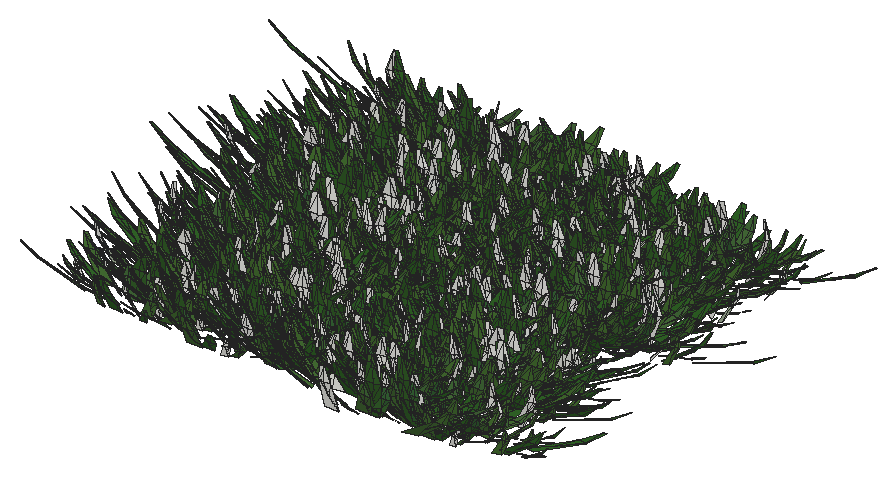
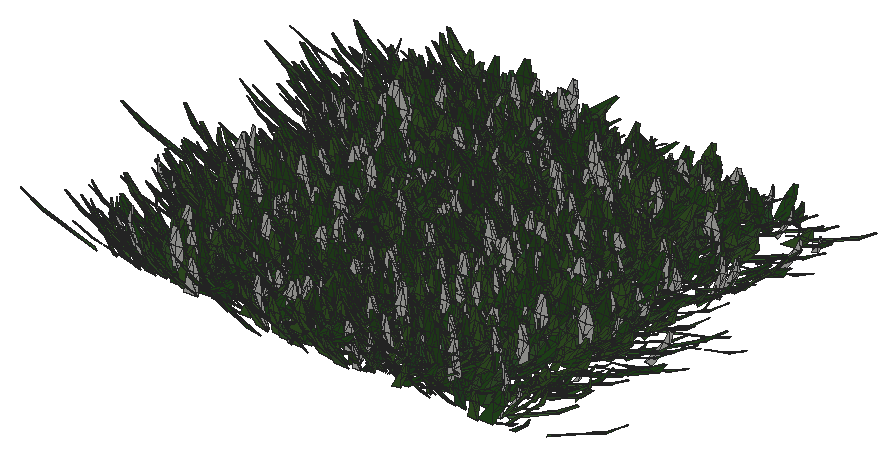
# SketchUp Ruby script. Lengths in inches.
U = 1.inch
M = Sketchup.active_model
def pt(a) = Geom::Point3d.new(a.map { |v| v * U })
def face(e, loops, mat)
  f = e.add_face(loops[0].map { |a| pt(a) })
  loops[1..].each { |l| e.add_face(l.map { |a| pt(a) }).erase! }
  f.material = f.back_material = mat if mat
  f
end
# faces: each face lists its corners as indices into pts; further lists are holes
def faces(e, pts, list, mat = nil) = list.each { |f| face(e, (f[0].is_a?(Array) ? f : [f]).map { |l| l.map { |i| pts[i] } }, mat) }
# xy, xz, yz: faces in a plane at the given z, y or x. An outline is a flat list of corners, or four numbers for a rectangle; further outlines are holes
def ring(l) = l.size == 4 ? [[l[0], l[1]], [l[2], l[1]], [l[2], l[3]], [l[0], l[3]]] : l.each_slice(2).to_a
def flat(e, list, mat, &to3) = list.each { |f| face(e, (f[0].is_a?(Array) ? f : [f]).map { |l| ring(l).map { |u, v| to3.(u, v) } }, mat) }
def xy(e, z, list, mat = nil) = flat(e, list, mat) { |x, y| [x, y, z] }
def xz(e, y, list, mat = nil) = flat(e, list, mat) { |x, z| [x, y, z] }
def yz(e, x, list, mat = nil) = flat(e, list, mat) { |y, z| [x, y, z] }
def lines(e, pts, list) = list.each { |a, b| e.add_line(pt(pts[a]), pt(pts[b])) }
# prism: a flat outline (further loops are holes) pulled along v
def prism(e, loops, v, mat = nil)
  f = face(e, loops, mat); d = Geom::Vector3d.new(v.map { |x| x * U })
  f.pushpull(f.normal.samedirection?(d) ? d.length : -d.length)
end
def box(e, o, s, mat = nil) = prism(e, [[o, [o[0] + s[0], o[1], o[2]], [o[0] + s[0], o[1] + s[1], o[2]], [o[0], o[1] + s[1], o[2]]]], [0, 0, s[2]], mat)
def at(x, y, z, deg = 0) = Geom::Transformation.translation(pt([x, y, z])) * Geom::Transformation.rotation(ORIGIN, Z_AXIS, deg.degrees)
def axes(o, x, y, z) = Geom::Transformation.new([*x, 0, *y, 0, *z, 0, *pt(o).to_a, 1])
def part(name) = M.definitions.add(name)
# library, detail: a bought-in or finely detailed component or shape, given as its bounding box
def library(name, o, s) = part(name).tap { |d| box(d.entities, o, s) }
def detail(e, o, s) = box(e.add_group.entities, o, s)
def put(e, d, t, mat = nil) = e.add_instance(d, t).tap { |i| i.material = mat if mat }
def group(e, t, mat = nil) = e.add_group.tap { |g| g.transformation = t; g.material = mat if mat }.entities
root = M.entities
M.materials.add("Material10").color = [48, 100, 38]
M.materials.add("Material3").color = [68, 110, 58]
M.materials.add("Material4").color = [48, 90, 38]
M.materials.add("Material5").color = [68, 110, 48]
M.materials.add("Material6").color = [48, 90, 48]
M.materials.add("Material7").color = [58, 110, 58]
M.materials.add("Material8").color = [58, 90, 38]
M.materials.add("Material9").color = [68, 100, 58]
c1 = part("grass00")
p = [[-0.6875,0.15,0],[-0.56,0.08,5.52],[-0.04,0.03,2.76],[0.48,-0.02,0],[0.35,-0.02,5.52],[-0.1,-0.14,5.52],
  [-0.12,0.65,8.37],[-0.42,0.65,8.37]]
faces(c1.entities,p,[[0,1,2,3],[3,2,4],[1,5,2],[5,4,2],[1,6,5],[4,5,6],[7,6,1]])
c2 = part("Group16\#1")
put(c2.entities,c1,axes([1.44,-0.61,-0.01],[0.05352,0.12609,0],[-0.10704,0.04543,0.07239],[0.06664,-0.02828,0.11628]),"Material6")
put(c2.entities,c1,axes([0.76,-0.15,-0.01],[0.04676,0.24062,0],[-0.23162,0.04501,0.06642],[0.0652,-0.01267,0.23595]),"Material3")
put(c2.entities,c1,axes([0.79,0.01,-0.01],[-0.00606,0.34651,0],[-0.34381,-0.00602,0.0432],[0.04319,0.00076,0.34386]))
put(c2.entities,c1,axes([1,0.23,-0.01],[-0.07192,0.31144,0],[-0.28722,-0.06632,0.1236],[0.12043,0.02781,0.29478]),"Material5")
put(c2.entities,c1,axes([1.66,0.77,-0.01],[-0.13828,0.29651,0],[-0.21551,-0.1005,0.22471],[0.20365,0.09498,0.23779]),"Material10")
put(c2.entities,c1,axes([0.6875,0.52,-0.01],[-0.18126,0.24051,0],[-0.22746,-0.17142,0.09788],[0.07817,0.05891,0.28481]),"Material5")
put(c2.entities,c1,axes([0.68,0.78,-0.01],[-0.215,0.18688,0],[-0.12385,-0.14248,0.21334],[0.13995,0.16101,0.18878]),"Material3")
put(c2.entities,c1,axes([0.56,1,-0.01],[-0.13756,0.07624,0],[-0.06159,-0.11112,0.0927],[0.04494,0.08108,0.12705]),"Material5")
put(c2.entities,c1,axes([0.2,0.64,-0.01],[-0.23729,0.07254,0],[-0.05711,-0.18681,0.153],[0.04473,0.14632,0.19535]),"Material10")
put(c2.entities,c1,axes([0.0625,0.72,-0.01],[-0.28874,0.02525,0],[-0.02179,-0.24916,0.14647],[0.01276,0.14591,0.25012]),"Material3")
put(c2.entities,c1,axes([-0.08,0.62,-0.01],[-0.34089,-0.04187,0],[0.03255,-0.26504,0.216],[-0.02633,0.21439,0.26703]),"Material10")
put(c2.entities,c1,axes([-0.34,0.98,-0.01],[-0.14314,-0.0493,0],[0.04397,-0.12769,0.06843],[-0.02228,0.0647,0.13505]),"Material10")
put(c2.entities,c1,axes([-0.87,1.45,-0.01],[-0.23488,-0.14114,0],[0.13761,-0.22901,0.06087],[-0.03135,0.05217,0.26717]))
put(c2.entities,c1,axes([-0.72,0.77,-0.01],[-0.14208,-0.13251,0],[0.07209,-0.0773,0.16301],[-0.11118,0.11922,0.1057]),"Material10")
put(c2.entities,c1,axes([-0.62,0.43,-0.01],[-0.14845,-0.21203,0],[0.18654,-0.13061,0.12304],[-0.10079,0.07057,0.22772]),"Material3")
put(c2.entities,c1,axes([-0.68,0.29,-0.01],[-0.13639,-0.32136,0],[0.31723,-0.13464,0.05579],[-0.05136,0.0218,0.34462]),"Material4")
put(c2.entities,c1,axes([-0.64,0.125,-0.01],[-0.0458,-0.23569,0],[0.22124,-0.043,0.08276],[-0.08124,0.01579,0.22538]),"Material7")
put(c2.entities,c1,axes([-1.6,-0.03,-0.01],[0.00576,-0.32897,0],[0.27526,0.00482,0.18018],[-0.18015,-0.00315,0.2753]),"Material5")
put(c2.entities,c1,axes([-1.36,-0.31,-0.01],[0.05718,-0.24765,0],[0.18172,0.04196,0.17267],[-0.16825,-0.03885,0.1865]),"Material10")
put(c2.entities,c1,axes([-1.54,-0.72,-0.01],[0.06537,-0.14017,0],[0.13555,0.06321,0.03939],[-0.0357,-0.01665,0.14956]))
put(c2.entities,c1,axes([-1.19,-0.9,-0.01],[0.09597,-0.12735,0],[0.11214,0.08451,0.07557],[-0.06035,-0.04548,0.14042]),"Material9")
put(c2.entities,c1,axes([-0.47,-0.54,-0.01],[0.11588,-0.10072,0],[0.0618,0.0711,0.12124],[-0.07953,-0.0915,0.0942]))
put(c2.entities,c1,axes([-0.47,-0.84,-0.01],[0.11927,-0.0661,0],[0.06603,0.11913,0.00646],[-0.00313,-0.00565,0.13621]),"Material5")
put(c2.entities,c1,axes([-0.38,-1.24,-0.01],[0.28037,-0.08571,0],[0.0618,0.20215,0.20315],[-0.05939,-0.19428,0.21139]),"Material9")
put(c2.entities,c1,axes([-0.06,-0.66,-0.01],[0.22719,-0.01987,0],[0.01247,0.14255,0.17758],[-0.01547,-0.17691,0.1431]),"Material8")
put(c2.entities,c1,axes([0.11,-0.89,-0.01],[0.14882,0.01828,0],[-0.01058,0.08611,0.12229],[0.01491,-0.12138,0.08676]),"Material6")
put(c2.entities,c1,axes([0.25,-0.72,-0.01],[0.20481,0.07053,0],[-0.06206,0.18022,0.10291],[0.03351,-0.0973,0.1906]),"Material6")
put(c2.entities,c1,axes([0.85,-1.42,-0.01],[0.16481,0.09904,0],[-0.09472,0.15762,0.05616],[0.02893,-0.04814,0.18389]),"Material5")
put(c2.entities,c1,axes([1.01,-1.09,-0.01],[0.21858,0.20385,0],[-0.17495,0.1876,0.15339],[0.10462,-0.11218,0.25652]),"Material10")
put(c2.entities,c1,axes([1.01,-0.71,-0.01],[0.08733,0.12473,0],[-0.06445,0.04512,0.13037],[0.1068,-0.07477,0.07867]),"Material6")
c3 = part("Group15\#1")
put(c3.entities,c2,at(0,0,0))
c4 = part("3darcstudiotree_grass00\#1")
put(c4.entities,c3,at(0,0,0))
put(root,c4,axes([888.96,967.25,0],[-1.13756,-1.10329,0],[4.36364,-0.2812,-0.01269],[0.0739,-0.00476,1.69312]))
put(root,c4,axes([887.47,959.43,0],[-1.05633,0.97001,0],[-4.93574,-0.33594,-0.06593],[-0.31871,-0.02169,1.60187]))
put(root,c4,axes([889.01,948.79,0],[-1.37062,-0.86535,0],[3.38403,-0.33499,-0.01359],[0.09291,-0.0092,1.67314]))
put(root,c4,axes([888.71,972.6,0],[-4.71082,0.41428,0],[-1.209,-0.85923,-0.00518],[-0.01407,-0.01,1.86492]))
put(root,c4,axes([888.36,953.27,0],[-3.26227,0.95653,0],[-3.0473,-0.64955,-0.01811],[-0.0716,-0.01526,1.30017]))
put(root,c4,axes([888.56,934.67,0],[2.69465,-0.83089,0],[3.37548,0.68418,-0.02965],[0.1163,0.02357,1.3715]))
put(root,c4,axes([890.17,957.41,0],[-4.67486,-0.01007,0],[0.0413,-1.19802,-0.00939],[0.00051,-0.01491,1.9024]))
put(root,c4,axes([889.79,965.56,0],[2.36561,-1.09039,0],[3.75477,0.50912,-0.01711],[0.08085,0.01096,1.43496]))
put(root,c4,axes([888.65,945.09,0],[3.54618,0.29573,0],[-1.39586,1.04613,-0.00681],[-0.0149,0.01117,1.90695]))
put(root,c4,axes([890.66,956.25,0],[0.13363,-1.19424,0],[4.75685,0.03327,-0.00421],[0.02569,0.00018,1.81536]))
put(root,c4,axes([889,943.72,0],[3.3147,0.39945,0],[-1.62402,0.84226,-0.04063],[-0.11562,0.05996,1.53169]))
put(root,c4,axes([889.14,940.41,0],[-0.8661,0.95762,0],[-4.99229,-0.2822,-0.04071],[-0.17859,-0.0101,1.43871]))
put(root,c4,axes([889.63,961.95,0],[-1.64669,0.8129,0],[-3.86386,-0.48919,-0.03106],[-0.13559,-0.01717,1.32443]))
put(root,c4,axes([890.23,960.95,0],[-0.66417,1.24214,0],[-3.94693,-0.1319,-0.04319],[-0.32199,-0.01076,1.87209]))
put(root,c4,axes([891.4,969.1875,0],[-2.88434,-1.08053,0],[3.30861,-0.55199,-0.04802],[0.27291,-0.04553,1.69851]))
put(root,c4,axes([891.54,968.69,0],[-2.43926,-0.75546,0],[3.00839,-0.6071,-0.02577],[0.12993,-0.02622,1.56591]))
put(root,c4,axes([891.68,954.41,0],[1.40965,-1.22459,0],[4.89499,0.35217,-0.04991],[0.29274,0.02106,1.94306]))
put(root,c4,axes([890.71,947.16,0],[4.02811,0.14495,0],[-0.62755,1.08997,-0.04848],[-0.03789,0.0658,1.51023]))
put(root,c4,axes([891.92,951.83,0],[1.97657,-1.09478,0],[4.53961,0.51226,-0.03311],[0.18515,0.02089,1.9099]))
put(root,c4,axes([891.75,963.5,0],[3.73189,-0.79039,0],[3.05525,0.9016,-0.02128],[0.07472,0.02205,1.60475]))
put(root,c4,axes([891.03,970.89,0],[3.02072,0.55371,0],[-2.49309,0.85005,-0.01003],[-0.03081,0.0105,1.36834]))
put(root,c4,axes([891.85,936.17,0],[-0.05036,0.9122,0],[-4.03492,-0.01392,-0.02407],[-0.14251,-0.00049,1.49365]))
put(root,c4,axes([894.64,941.17,0],[0.09023,-0.92419,0],[3.99755,0.02439,-0.00377],[0.02513,0.00015,1.66719]))
put(root,c4,axes([894.16,954.03,0],[-2.09892,1.15231,0],[-3.29486,-0.3751,-0.04508],[-0.24035,-0.02736,1.32557]))
put(root,c4,axes([893.93,959.11,0],[4.49325,-0.21308,0],[0.91825,1.21019,-0.00778],[0.00669,0.00882,1.42033]))
put(root,c4,axes([894.36,947.36,0],[-2.22405,0.97958,0],[-4.34161,-0.61608,-0.03094],[-0.11665,-0.01655,1.35284]))
put(root,c4,axes([894.16,948.26,0],[4.35501,-0.07003,0],[0.31999,1.24382,-0.04097],[0.01403,0.05455,1.66267]))
put(root,c4,axes([894.89,952.55,0],[3.24444,-0.662,0],[2.42795,0.74371,-0.03627],[0.18046,0.05528,1.88825]))
put(root,c4,axes([896.16,942.22,0],[-2.89851,-0.94467,0],[3.35055,-0.64252,-0.03114],[0.17556,-0.03367,1.87535]))
put(root,c4,axes([895.52,969.3125,0],[3.0338,-0.77588,0],[3.0604,0.74791,-0.00015],[0.00078,0.00019,1.98495]))
put(root,c4,axes([894.55,944.25,0],[1.49753,0.88815,0],[-4.28846,0.45193,-0.04214],[-0.25848,0.02724,1.93625]))
put(root,c4,axes([896.6,957.35,0],[-0.51089,-1.13336,0],[4.16419,-0.11732,-0.02839],[0.14199,-0.004,1.31807]))
put(root,c4,axes([896.71,961.98,0],[-2.45945,-0.81694,0],[3.01218,-0.56677,-0.02546],[0.16778,-0.03157,1.94365]))
put(root,c4,axes([897.37,968.51,0],[-3.46196,-0.96436,0],[3.51371,-0.78837,-0.02493],[0.09006,-0.02021,1.43253]))
put(root,c4,axes([897.08,971.33,0],[-4.50327,-0.2714,0],[0.9427,-0.97764,-0.01967],[0.02949,-0.03058,1.60841]))
put(root,c4,axes([896.39,950.2,0],[-2.75992,0.94196,0],[-2.97534,-0.54485,-0.02032],[-0.11782,-0.02158,1.65635]))
put(root,c4,axes([897.09,936.4,0],[-4.30976,0.17306,0],[-0.69895,-1.08789,-0.04907],[-0.04617,-0.07186,1.63442]))
put(root,c4,axes([896.65,963.8,0],[1.62415,-0.82572,0],[3.47351,0.42701,-0.04022],[0.29805,0.03664,1.99791]))
put(root,c4,axes([895.72,934.46,0],[-0.21475,1.16093,0],[-4.31768,-0.04992,-0.00948],[-0.04784,-0.00055,1.36423]))
put(root,c4,axes([897.65,964.99,0],[-1.92009,-1.06648,0],[4.1428,-0.46617,-0.04331],[0.26264,-0.02955,1.88835]))
put(root,c4,axes([897.81,966.83,0],[-1.61898,-1.19321,0],[3.76246,-0.31906,-0.01224],[0.0924,-0.00784,1.97883]))
put(root,c4,axes([895.86,951.46,0],[0.9763,1.20206,0],[-4.96643,0.2521,-0.02679],[-0.14937,0.00758,1.80175]))
put(root,c4,axes([896.5,937.56,0],[3.61009,-0.1138,0],[0.57858,1.14719,-0.05027],[0.03392,0.06725,1.55905]))
put(root,c4,axes([895.86,960.38,0],[2.01763,0.79304,0],[-4.00397,0.63667,-0.00074],[-0.00407,0.00065,1.93092]))
put(root,c4,axes([897.42,945.71,0],[3.2052,-0.51026,0],[2.09643,0.82305,-0.0345],[0.14052,0.05517,1.8497]))
put(root,c4,axes([897.64,939.68,0],[0.11052,0.97112,0],[-4.47276,0.03182,-0.02239],[-0.14712,0.00105,1.83839]))
put(root,c4,axes([897.73,955.78,0],[-0.51157,1.00032,0],[-4.92552,-0.15743,-0.0277],[-0.16641,-0.00532,1.87956]))
put(root,c4,axes([899.95,948.87,0],[-2.88645,-0.88877,0],[3.86578,-0.78468,-0.02494],[0.12186,-0.02474,1.95866]))
put(root,c4,axes([899.91,972.5625,0],[-4.37,-0.28374,0],[1.17026,-1.12647,-0.00758],[0.01125,-0.01083,1.7185]))
put(root,c4,axes([899.61,955.97,0],[-0.06579,-0.95839,0],[4.48291,-0.01923,-0.0405],[0.2731,-0.00117,1.89003]))
put(root,c4,axes([900.04,960.89,0],[-1.52084,-1.07462,0],[3.90834,-0.3457,-0.03351],[0.20602,-0.01822,1.68972]))
put(root,c4,axes([900.71,968,0],[-1.03944,-1.24074,0],[4.69727,-0.24595,-0.02019],[0.11188,-0.00586,1.69814]))
put(root,c4,axes([900.53,971.7,0],[-0.98612,-1.22055,0],[4.4455,-0.22448,-0.03802],[0.23503,-0.01187,1.78771]))
put(root,c4,axes([900.89,950.46,0],[-3.13643,-0.44743,0],[1.98712,-0.87059,-0.04344],[0.16835,-0.07376,1.9596]))
put(root,c4,axes([901.15,942.05,0],[-1.81933,-1.05694,0],[4.48084,-0.48206,-0.04688],[0.23644,-0.02544,1.67419]))
put(root,c4,axes([901.08,946.57,0],[-3.96294,0.68936,0],[-2.37942,-0.85491,-0.01001],[-0.0292,-0.01049,1.32974]))
put(root,c4,axes([902.18,954.55,0],[-0.37875,-1.01008,0],[4.48858,-0.10519,-0.00863],[0.04422,-0.00104,1.44957]))
put(root,c4,axes([902.82,945.42,0],[-1.70482,-1.13891,0],[4.74643,-0.44405,-0.05081],[0.22443,-0.021,1.49393]))
put(root,c4,axes([901.28,952.8,0],[4.79231,-0.42159,0],[1.43855,1.02203,-0.0057],[0.01193,0.00848,1.70987]))
put(root,c4,axes([902.91,965.25,0],[-0.51771,-1.03917,0],[4.88499,-0.15211,-0.06365],[0.38906,-0.01211,1.89522]))
put(root,c4,axes([902.46,962.49,0],[2.41645,-0.95234,0],[3.1357,0.49728,-0.01781],[0.0973,0.01543,1.50117]))
put(root,c4,axes([902.07,970.18,0],[3.95263,-0.39442,0],[1.50714,0.94398,-0.02611],[0.05477,0.0343,1.43783]))
put(root,c4,axes([903.37,937.49,0],[-4.30049,-0.11953,0],[0.50316,-1.13147,-0.05312],[0.03445,-0.07747,1.67036]))
put(root,c4,axes([902.17,936.09,0],[4.68959,-0.46091,0],[1.44891,0.92138,-0.00849],[0.02258,0.01436,1.79934]))
put(root,c4,axes([903.58,958.95,0],[0.57687,-1.07494,0],[3.69634,0.12398,-0.00096],[0.00701,0.00024,1.71349]))
put(root,c4,axes([903.55,957.58,0],[-4.14654,0.02565,0],[-0.12263,-1.23885,-0.01248],[-0.00137,-0.01382,1.37214]))
put(root,c4,axes([903.79,966.93,0],[-3.83685,0.38096,0],[-1.50034,-0.94442,-0.04199],[-0.1028,-0.06471,1.68502]))
put(root,c4,axes([903.61,951.57,0],[-4.14844,0.73182,0],[-2.28116,-0.8082,0],[-0.00002,-0.00001,1.91868]))
put(root,c4,axes([902.8,935.1,0],[3.44069,0.27197,0],[-1.2898,1.01983,-0.04459],[-0.0839,0.06634,1.66873]))
put(root,c4,axes([904.11,963.45,0],[-4.43528,0.66628,0],[-1.93205,-0.80382,-0.02116],[-0.06942,-0.02888,1.49339]))
put(root,c4,axes([903.78,939.625,0],[-2.3482,0.69512,0],[-3.39481,-0.71676,-0.03207],[-0.17565,-0.03709,1.99077]))
put(root,c4,axes([903.99,941.03,0],[-3.32313,0.94443,0],[-3.84247,-0.84503,-0.06393],[-0.21081,-0.04636,1.40472]))
put(root,c4,axes([903.8,943.51,0],[4.99296,-0.12006,0],[0.49346,1.28259,-0.06081],[0.02614,0.06795,1.44654]))
put(root,c4,axes([905.84,954.1,0],[-0.04021,-0.94349,0],[5.12162,-0.01364,-0.05216],[0.22205,-0.00059,1.36288]))
put(root,c4,axes([905.95,944.01,0],[0.15214,-1.25594,0],[4.48063,0.03392,-0.01983],[0.10676,0.00081,1.50947]))
put(root,c4,axes([906.23,966.86,0],[-0.76774,-1.16095,0],[4.52934,-0.18721,-0.0168],[0.08958,-0.0037,1.55067]))
put(root,c4,axes([906.38,946.78,0],[-4.11234,-0.7945,0],[2.93722,-0.95019,-0.06061],[0.1773,-0.05736,1.43628]))
put(root,c4,axes([905.86,955.61,0],[-0.59166,-1.13858,0],[3.64186,-0.11828,-0.04034],[0.25705,-0.00835,1.47504]))
put(root,c4,axes([906.12,952.71,0],[-3.92438,0.31948,0],[-1.16946,-0.89782,-0.04555],[-0.09619,-0.07385,1.60995]))
put(root,c4,axes([906.63,937.57,0],[-4.2338,0.39742,0],[-1.47473,-0.9819,-0.01194],[-0.02743,-0.01826,1.71307]))
put(root,c4,axes([906.85,942.74,0],[-3.93577,0.74976,0],[-2.5237,-0.82799,-0.04347],[-0.16838,-0.05524,1.66314]))
put(root,c4,axes([907.71,935.24,0],[-3.54943,-0.49503,0],[1.78138,-0.79829,-0.00653],[0.02016,-0.00904,1.4475]))
put(root,c4,axes([908.08,965.55,0],[-3.36621,-0.95264,0],[2.81846,-0.62245,-0.00245],[0.01476,-0.00326,1.8862]))
put(root,c4,axes([906.1875,969.66,0],[0.43598,1.04612,0],[-4.32547,0.11267,-0.02993],[-0.17694,0.00461,1.61572]))
put(root,c4,axes([906.29,951.22,0],[-0.51235,0.89086,0],[-4.17612,-0.15011,-0.00494],[-0.0262,-0.00094,1.4129]))
put(root,c4,axes([908.25,939.4,0],[0.5765,-1.16396,0],[4.70538,0.14566,-0.00236],[0.01265,0.00039,1.5989]))
put(root,c4,axes([906.85,967.93,0],[4.23792,-0.23922,0],[0.87195,0.96546,-0.03599],[0.04234,0.04688,1.32194]))
put(root,c4,axes([908.03,957.65,0],[-4.26388,0.42681,0],[-1.64791,-1.02893,-0.00598],[-0.01365,-0.00852,1.70205]))
put(root,c4,axes([907.1,940.51,0],[4.67345,-0.08796,0],[0.29357,0.97489,-0.02417],[0.01343,0.0446,1.80918]))
put(root,c4,axes([907.16,970.82,0],[0.19862,1.12263,0],[-4.23211,0.0468,-0.03464],[-0.20461,0.00226,1.56527]))
put(root,c4,axes([906.92,972.3,0],[2.93954,0.6812,0],[-3.37406,0.90999,-0.0132],[-0.04593,0.01239,1.58767]))
put(root,c4,axes([908.86,948.24,0],[-4.4154,0.08876,0],[-0.37121,-1.15413,-0.04274],[-0.0155,-0.04821,1.31001]))
put(root,c4,axes([909.23,958.82,0],[-2.79225,-0.78906,0],[3.01148,-0.66605,-0.02762],[0.13842,-0.03061,1.68176]))
put(root,c4,axes([907.36,949.66,0],[2.75191,0.75526,0],[-3.57518,0.81417,-0.05824],[-0.22433,0.05109,1.57486]))
put(root,c4,axes([908.64,961.83,0],[2.32702,-1.05964,0],[3.64306,0.50002,-0.02765],[0.14347,0.01969,1.53783]))
put(root,c4,axes([907.9,936.27,0],[2.82481,0.56439,0],[-2.40364,0.7519,-0.04441],[-0.20419,0.06387,1.772]))
put(root,c4,axes([908.91,963.38,0],[2.47739,-0.8352,0],[3.76427,0.69785,-0.03781],[0.14929,0.02768,1.4396]))
put(root,c4,axes([908,960.32,0],[0.70904,1.19285,0],[-3.93143,0.14606,-0.03328],[-0.20326,0.00755,1.53387]))
put(root,c4,axes([909.17,945.2,0],[1.81143,0.91865,0],[-4.40364,0.5427,-0.01549],[-0.06434,0.00793,1.42146]))
put(root,c4,axes([912.17,935.9375,0],[-2.19017,-0.8406,0],[3.99666,-0.65083,-0.00487],[0.02392,-0.0039,1.74651]))
put(root,c4,axes([911.93,970.2,0],[-4.47501,0.4091,0],[-1.26068,-0.86189,-0.04181],[-0.08597,-0.05877,1.37365]))
put(root,c4,axes([912.22,958.68,0],[1.03732,-1.10415,0],[4.61468,0.27096,-0.04288],[0.24016,0.0141,1.70449]))
put(root,c4,axes([912.44,937.86,0],[0.84131,-0.93334,0],[4.465,0.25155,-0.02216],[0.11535,0.0065,1.52603]))
put(root,c4,axes([913.14,963.21,0],[-4.69083,0.06991,0],[-0.27853,-1.16812,-0.00226],[-0.00086,-0.00362,1.87745]))
put(root,c4,axes([912.78,966.73,0],[1.83497,-0.94895,0],[3.86157,0.46669,-0.03335],[0.17925,0.02166,1.60043]))
put(root,c4,axes([913.45,944.05,0],[-0.52129,-1.09873,0],[4.55576,-0.13509,-0.02638],[0.13198,-0.00391,1.44452]))
put(root,c4,axes([912.85,933.38,0],[-3.80246,0.84843,0],[-3.3004,-0.92448,-0.01139],[-0.04326,-0.01212,1.76647]))
put(root,c4,axes([912.4,960.74,0],[4.54978,-0.41024,0],[1.68506,1.16802,-0.06016],[0.10033,0.06955,1.52593]))
put(root,c4,axes([912.68,950.01,0],[-1.83035,0.9083,0],[-3.79147,-0.47752,-0.03585],[-0.1914,-0.02411,1.58646]))
put(root,c4,axes([913.33,954.58,0],[-3.83368,0.65394,0],[-2.36906,-0.86802,-0.04776],[-0.17139,-0.0628,1.6727]))
put(root,c4,axes([912.62,948.82,0],[4.16884,-0.44191,0],[1.67994,0.9905,-0.02583],[0.06325,0.03729,1.68703]))
put(root,c4,axes([913.0625,968.3,0],[5.02787,-0.3126,0],[0.9305,0.9354,-0.00031],[0.00054,0.00054,1.72722]))
put(root,c4,axes([913.66,945.02,0],[3.79189,-0.60703,0],[2.47223,0.9652,-0.00312],[0.00888,0.00347,1.51309]))
put(root,c4,axes([913.25,947.14,0],[4.87895,-0.29762,0],[0.96688,0.99066,-0.01844],[0.03122,0.03199,1.82062]))
put(root,c4,axes([914.29,962.04,0],[2.31216,-0.81915,0],[3.42555,0.60431,-0.01427],[0.0583,0.01029,1.30992]))
put(root,c4,axes([914.39,940.62,0],[2.96673,-0.89554,0],[3.5792,0.74107,-0.01649],[0.07862,0.01628,1.79785]))
put(root,c4,axes([915.19,956.4,0],[-2.17941,-0.94456,0],[3.95832,-0.57082,-0.05686],[0.22617,-0.03262,1.31145]))
put(root,c4,axes([915.17,971.12,0],[-5.07724,0.11974,0],[-0.34282,-0.90851,-0.02738],[-0.01844,-0.04887,1.63584]))
put(root,c4,axes([914.82,953.14,0],[1.32432,-1.09589,0],[4.49114,0.3392,-0.03916],[0.2319,0.01751,1.81408]))
put(root,c4,axes([913.22,957.35,0],[2.43888,0.92157,0],[-4.2022,0.69505,-0.02773],[-0.11094,0.01835,1.51065]))
put(root,c4,axes([914.09,965.25,0],[0.35474,0.89706,0],[-4.2384,0.10475,-0.01511],[-0.11034,0.00273,1.95375]))
put(root,c4,axes([914.3,938.85,0],[3.6065,0.55096,0],[-2.61428,1.06954,-0.04231],[-0.13529,0.05535,1.92144]))
put(root,c4,axes([916.17,942.68,0],[-4.74317,0.13037,0],[-0.40737,-0.92635,-0.04038],[-0.03022,-0.06871,1.5952]))
put(root,c4,axes([915.79,934.93,0],[-2.66919,0.82783,0],[-2.98072,-0.60068,-0.02131],[-0.13141,-0.02648,1.8955]))
put(root,c4,axes([915.73,951.85,0],[-1.19355,0.89536,0],[-3.41467,-0.28449,-0.02384],[-0.1819,-0.01516,1.80943]))
put(root,c4,axes([917.8125,957.49,0],[0.34278,-0.91027,0],[3.93669,0.09265,-0.01523],[0.12213,0.00287,1.99019]))
put(root,c4,axes([918.42,938.85,0],[-3.72708,-0.77449,0],[2.33482,-0.70224,-0.01701],[0.09318,-0.02803,1.95649]))
put(root,c4,axes([918.8125,947.97,0],[-3.89564,-0.27559,0],[0.99686,-0.8807,-0.03071],[0.05069,-0.04478,1.38702]))
put(root,c4,axes([918.27,944.28,0],[1.68583,-0.81683,0],[4.11916,0.53134,-0.04957],[0.26252,0.03386,1.72633]))
put(root,c4,axes([918.79,965.41,0],[-0.13589,-1.00462,0],[3.6498,-0.03085,-0.02047],[0.14931,-0.00126,1.66543]))
put(root,c4,axes([918.49,942.58,0],[2.09408,-1.17299,0],[4.38498,0.48927,-0.04062],[0.22124,0.02469,1.79015]))
put(root,c4,axes([918.41,963.56,0],[-3.01773,0.80944,0],[-3.41595,-0.79595,-0.00031],[-0.00127,-0.0003,1.61707]))
put(root,c4,axes([918.34,947.31,0],[3.44538,-0.3202,0],[1.49096,1.00268,-0.02775],[0.06957,0.04678,1.92398]))
put(root,c4,axes([918.63,933.875,0],[-1.08515,0.9046,0],[-3.54235,-0.26559,-0.04553],[-0.24621,-0.01846,1.30482]))
put(root,c4,axes([919.87,953.3125,0],[-0.65047,-1.04109,0],[4.03064,-0.1574,-0.04759],[0.24886,-0.00972,1.34947]))
put(root,c4,axes([920.48,962.19,0],[-2.08423,-0.85727,0],[3.21957,-0.48922,-0.04312],[0.30054,-0.04567,1.92045]))
put(root,c4,axes([920.67,968.58,0],[-2.32935,-0.7629,0],[3.09102,-0.58986,-0.04177],[0.18704,-0.03569,1.36919]))
put(root,c4,axes([920.8,945.375,0],[1.57863,-1.11612,0],[3.5477,0.31361,-0.02361],[0.12493,0.01104,1.32009]))
put(root,c4,axes([919.74,966.97,0],[1.59781,1.17762,0],[-4.51681,0.38303,-0.04327],[-0.24194,0.02052,1.7601]))
put(root,c4,axes([919.96,958.875,0],[0.44983,1.23092,0],[-3.94694,0.09015,-0.02215],[-0.12679,0.0029,1.42375]))
put(root,c4,axes([921.25,961.08,0],[1.0564,-1.26283,0],[3.63785,0.1902,-0.01603],[0.10027,0.00524,1.48463]))
put(root,c4,axes([920.17,941.46,0],[-0.94273,1.27464,0],[-5.04874,-0.23338,-0.00297],[-0.01721,-0.0008,1.8915]))
put(root,c4,axes([920.5,970.71,0],[4.33399,-0.08203,0],[0.31572,1.04255,-0.04662],[0.02263,0.07473,1.68074]))
put(root,c4,axes([920.66,970.14,0],[-0.71459,1.01896,0],[-4.19391,-0.18382,-0.02601],[-0.15992,-0.00701,1.66111]))
put(root,c4,axes([920.09,936.35,0],[3.19575,0.75582,0],[-3.09164,0.817,-0.00432],[-0.01514,0.004,1.43292]))
put(root,c4,axes([921.47,955.96,0],[3.81417,-0.56994,0],[2.46568,1.03131,-0.05659],[0.15929,0.06663,1.64805]))
put(root,c4,axes([920.87,934.75,0],[4.81538,0.36393,0],[-1.10544,0.91418,-0.04581],[-0.0874,0.07228,1.57403]))
put(root,c4,axes([920.84,954.7,0],[3.74971,0.70366,0],[-2.74434,0.91401,-0.02233],[-0.09238,0.03077,1.9689]))
